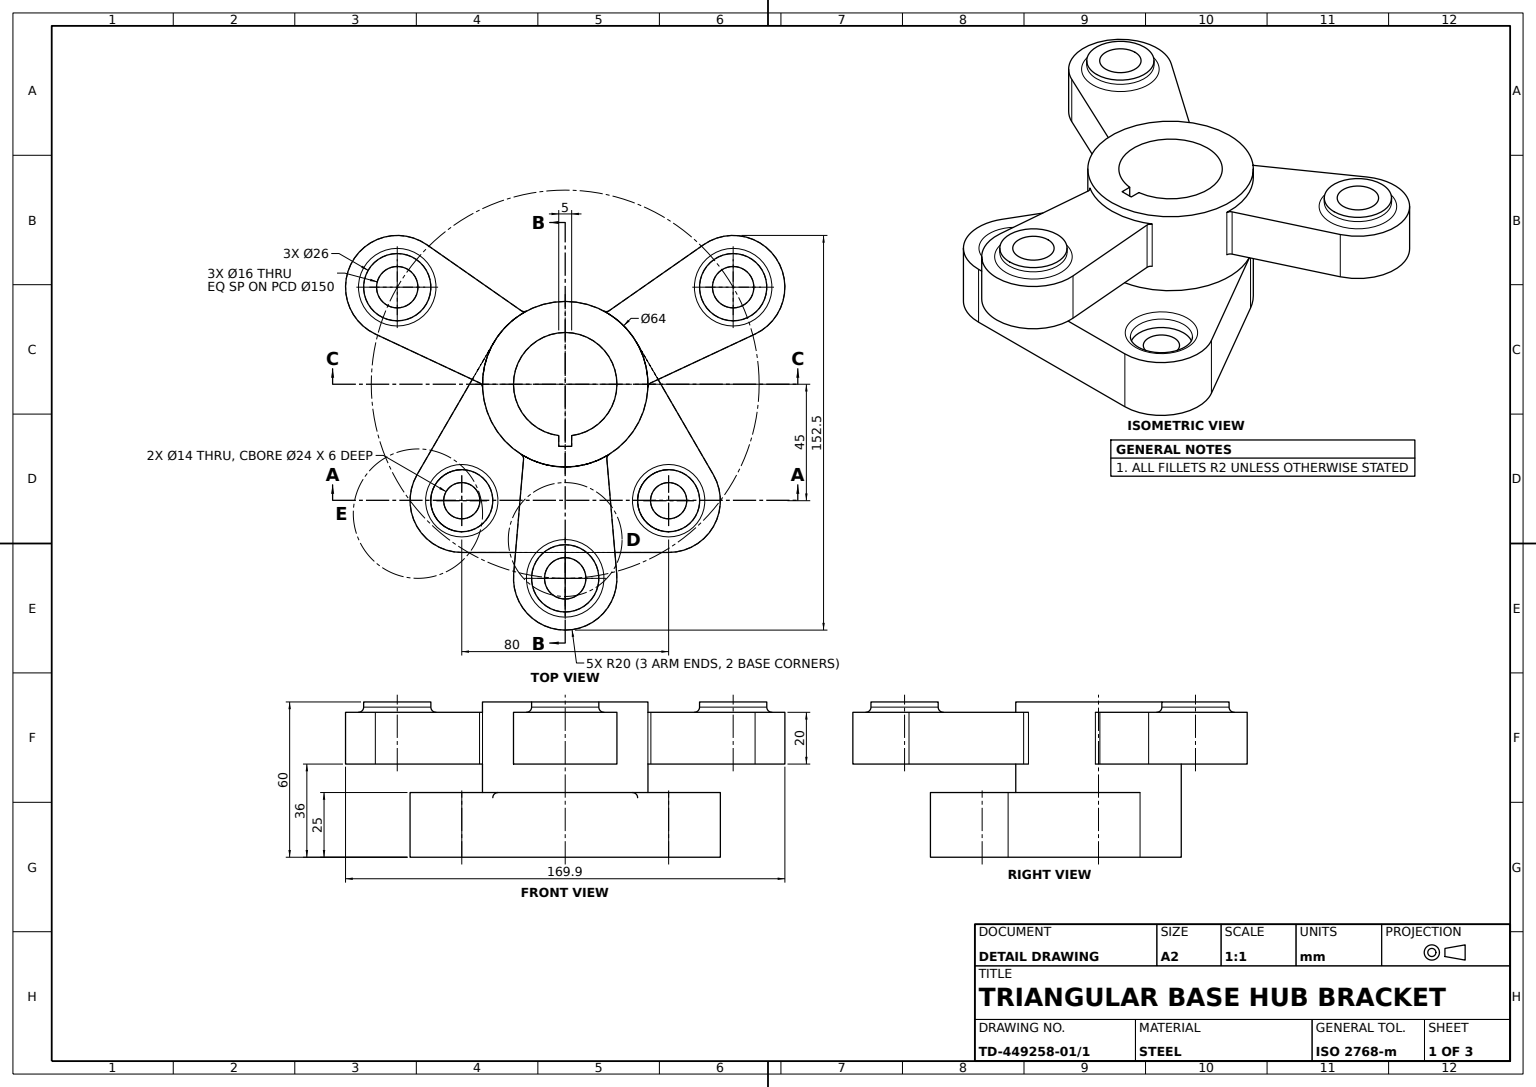
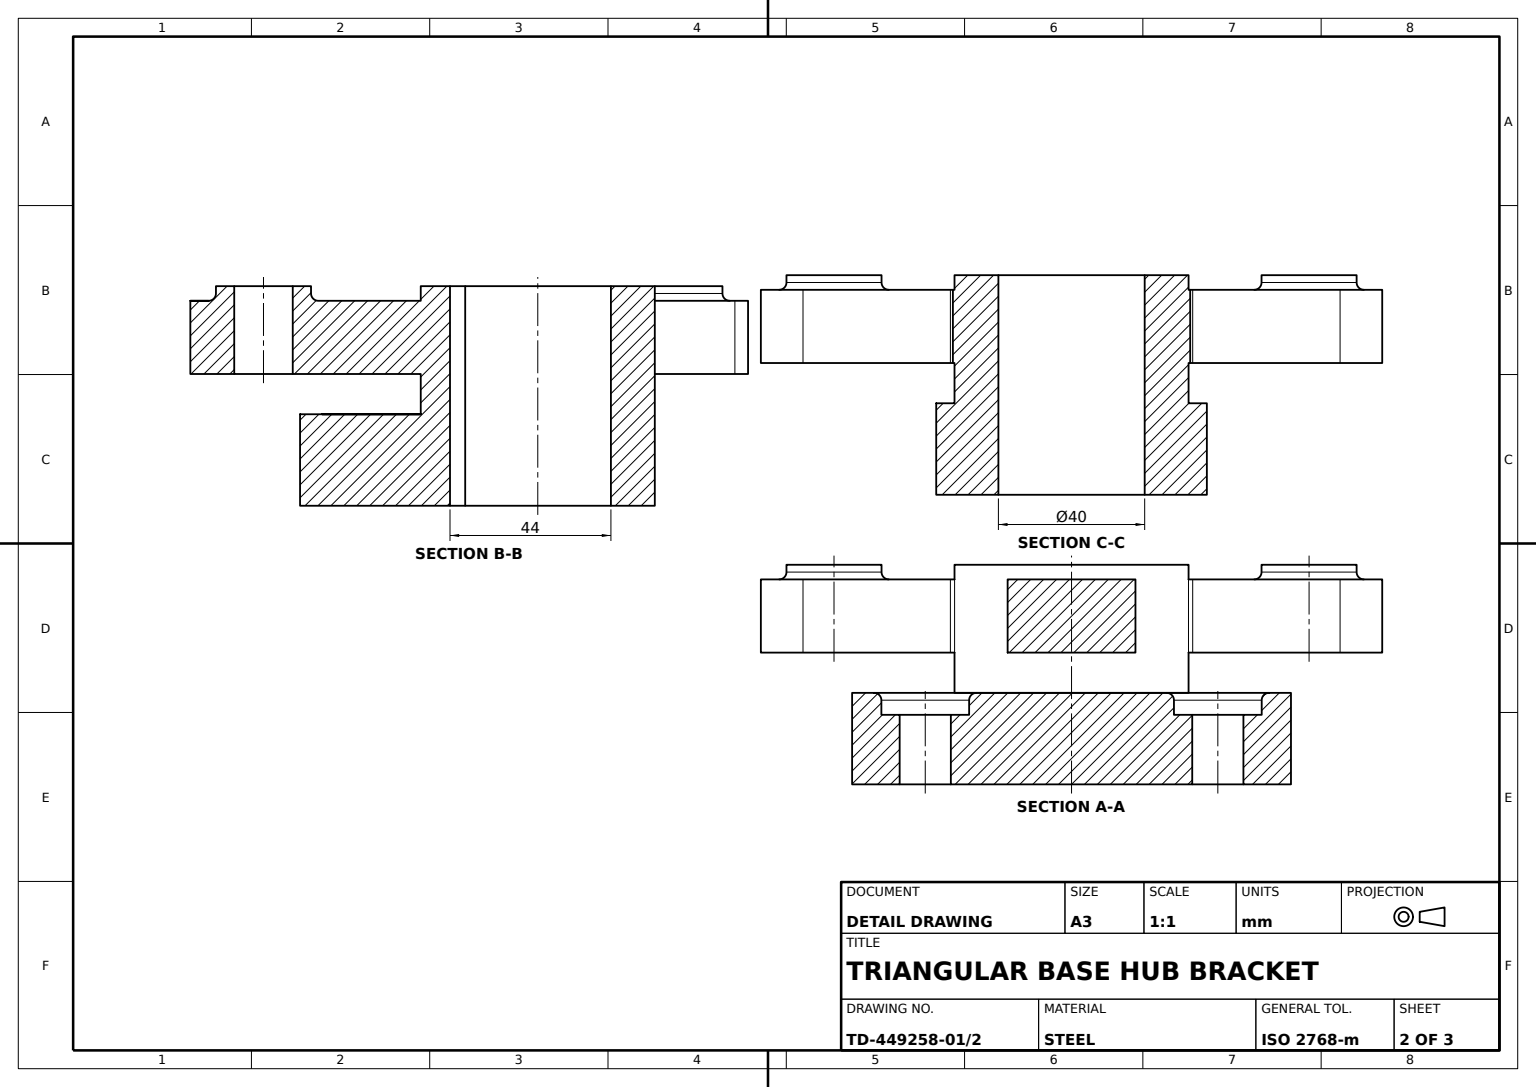
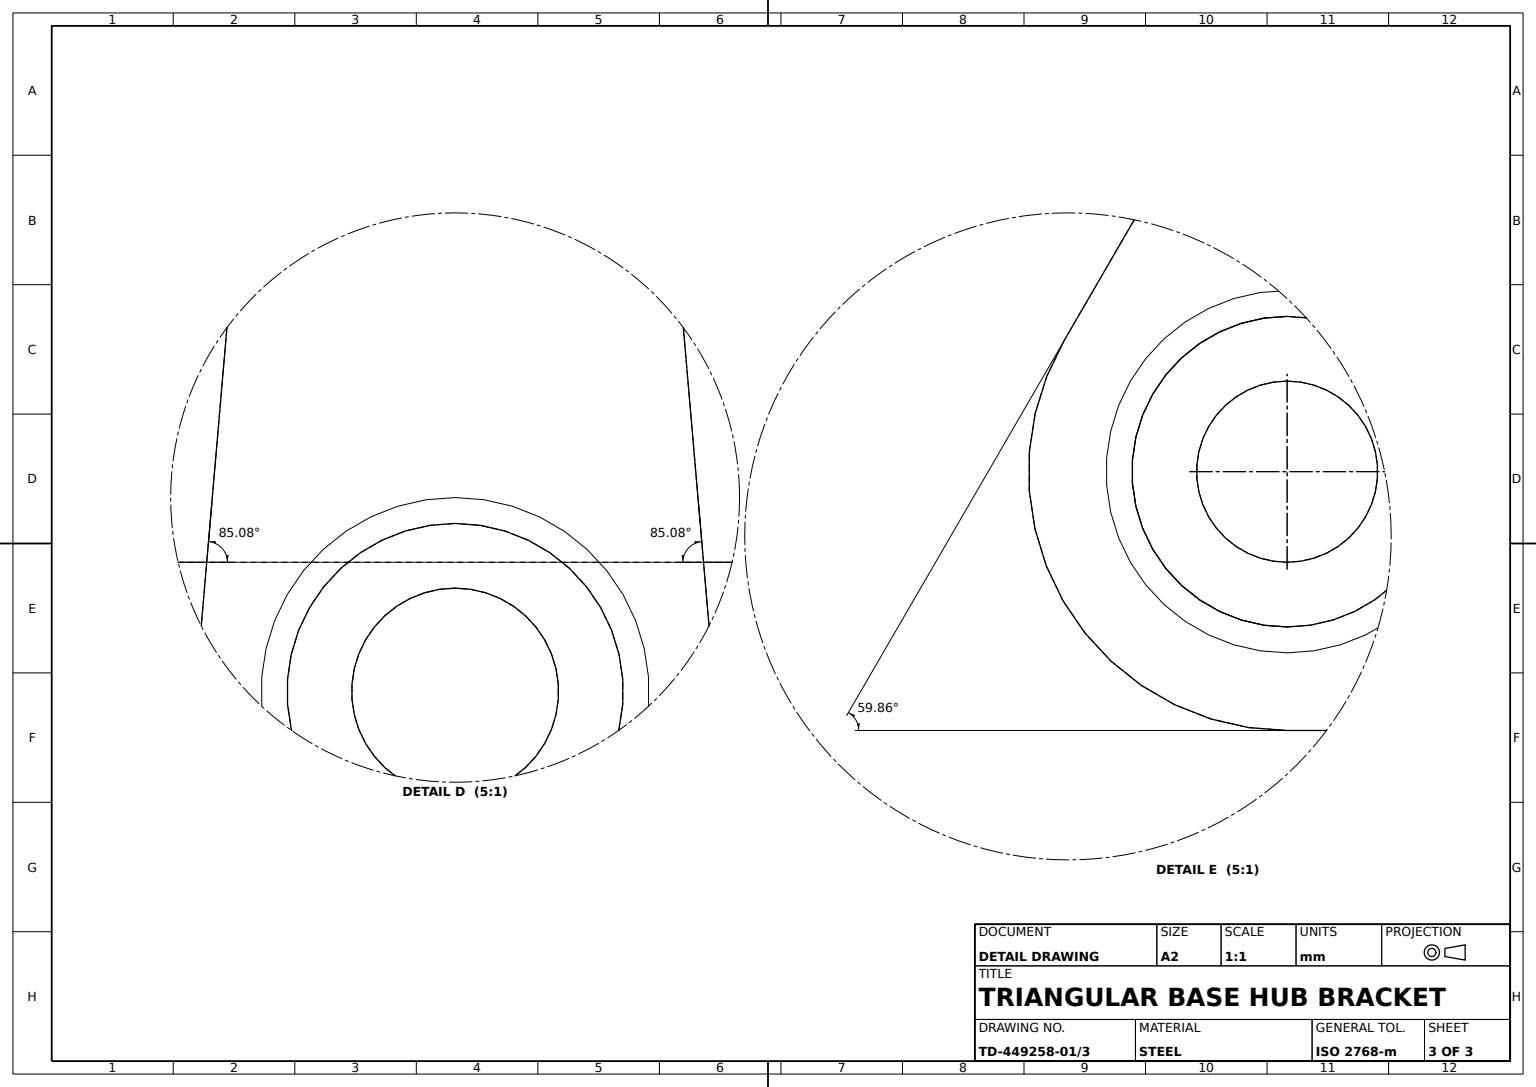
solid
v1 (73.428232,36,-19.385037)
v2 (73.428232,56,-19.385037)
e1 v1 v2 LINE
v3 (33.128128,56,-0.527872)
e2 v3 v2 LINE
v4 (33.128128,36,-0.527872)
e3 v3 v4 LINE
e4 v4 v1 LINE
face PLANE(AX(P(5.747849,36,12.283868),D(0.423816334,0,0.905748152),D(0.905748152,0,-0.423816334))) [e1 -e2 e3 e4]
v5 (-33.128128,36,-0.527872)
v6 (-73.428232,36,-19.385037)
e5 v5 v6 LINE
v7 (-33.128128,56,-0.527872)
e6 v5 v7 LINE
v8 (-73.428232,56,-19.385037)
e7 v7 v8 LINE
e8 v6 v8 LINE
face PLANE(AX(P(-5.747849,36,12.283868),D(0.423816334,0,-0.905748152),D(-0.905748152,0,-0.423816334))) rev [-e5 e6 e7 -e8]
v9 (-2.5,60,24)
v10 (-2.5,0,24)
e9 v9 v10 LINE
v11 (2.5,60,24)
e10 v11 v9 LINE
v12 (2.5,0,24)
e11 v11 v12 LINE
e12 v10 v12 LINE
face PLANE(AX(P(2.5,60,24),D(0,0,1),D(1,0,0))) rev [-e9 -e10 e11 -e12]
v13 (64.951905,58,-50.5)
v14 (64.951905,58,-24.5)
e13 v13 v14 CIRCLE(AX(P(64.951905,58,-37.5),D(0,1,0),D(0,0,1)),13)
v15 (64.951905,56,-52.5)
e14 v13 v15 CIRCLE(AX(P(64.951905,58,-52.5),D(1,0,0),D(0,0,-1)),2)
v16 (64.951905,56,-22.5)
e15 v16 v15 CIRCLE(AX(P(64.951905,56,-37.5),D(0,-1,0),D(0,0,1)),15)
e16 v14 v16 CIRCLE(AX(P(64.951905,58,-22.5),D(-1,0,0),D(0,0,1)),2)
face TORUS(AX(P(64.951905,58,-37.5),D(0,1,0),D(0,0,1)),15,2) rev [-e13 e14 -e15 -e16]
v17 (-64.951905,58,-24.5)
v18 (-64.951905,56,-22.5)
e17 v17 v18 CIRCLE(AX(P(-64.951905,58,-22.5),D(-1,0,0),D(0,0,1)),2)
v19 (-64.951905,58,-50.5)
e18 v19 v17 CIRCLE(AX(P(-64.951905,58,-37.5),D(0,1,0),D(0,0,1)),13)
v20 (-64.951905,56,-52.5)
e19 v19 v20 CIRCLE(AX(P(-64.951905,58,-52.5),D(1,0,0),D(0,0,-1)),2)
e20 v18 v20 CIRCLE(AX(P(-64.951905,56,-37.5),D(0,-1,0),D(0,0,1)),15)
face TORUS(AX(P(-64.951905,58,-37.5),D(0,1,0),D(0,0,1)),15,2) rev [-e17 -e18 e19 -e20]
v21 (0,0,-20)
v22 (-2.5,0,19.843135)
e21 v21 v22 CIRCLE(AX(P(0,0,0),D(0,1,0),D(0,0,1)),20)
v23 (0,60,-20)
e22 v23 v21 LINE
v24 (-2.5,60,19.843135)
e23 v23 v24 CIRCLE(AX(P(0,60,0),D(0,1,0),D(0,0,1)),20)
e24 v24 v22 LINE
face CYL(AX(P(0,60,0),D(0,-1,0),D(0,0,-1)),20) rev [-e21 -e22 e23 e24]
v25 (64.951905,36,-29.5)
v26 (64.951905,36,-45.5)
e25 v25 v26 CIRCLE(AX(P(64.951905,36,-37.5),D(0,1,0),D(0,0,1)),8)
e26 v26 v25 CIRCLE(AX(P(64.951905,36,-37.5),D(0,1,0),D(0,0,1)),8)
v27 (31.977186,36,1.208117)
e27 v4 v27 CIRCLE(AX(P(33.975761,36,1.283624),D(0,1,0),D(0,0,1)),2)
v28 (14.942333,36,-28.297114)
e28 v27 v28 CIRCLE(AX(P(0,36,0),D(0,1,0),D(0,0,1)),32)
v29 (17.021214,36,-28.425864)
e29 v28 v29 CIRCLE(AX(P(15.876229,36,-30.065684),D(0,1,0),D(0,0,1)),2)
v30 (53.50205,36,-53.898196)
e30 v29 v30 LINE
e31 v1 v30 CIRCLE(AX(P(64.951905,36,-37.5),D(0,1,0),D(0,0,1)),20)
face PLANE(AX(P(0,36,0),D(0,1,0),D(0,0,1))) rev [e25 e26] [e27 e28 e29 e30 -e31 -e4]
v31 (64.951905,60,-50.5)
v32 (64.951905,60,-24.5)
e32 v31 v32 CIRCLE(AX(P(64.951905,60,-37.5),D(0,1,0),D(0,0,1)),13)
e33 v32 v31 CIRCLE(AX(P(64.951905,60,-37.5),D(0,1,0),D(0,0,1)),13)
v33 (64.951905,60,-29.5)
v34 (64.951905,60,-45.5)
e34 v33 v34 CIRCLE(AX(P(64.951905,60,-37.5),D(0,1,0),D(0,0,1)),8)
e35 v34 v33 CIRCLE(AX(P(64.951905,60,-37.5),D(0,1,0),D(0,0,1)),8)
face PLANE(AX(P(0,60,0),D(0,1,0),D(0,0,1))) [e32 e33] [-e34 -e35]
v35 (0,36,83)
v36 (0,36,67)
e36 v35 v36 CIRCLE(AX(P(0,36,75),D(0,1,0),D(-0.866025404,0,-0.5)),8)
v37 (0,60,83)
e37 v35 v37 LINE
v38 (0,60,67)
e38 v37 v38 CIRCLE(AX(P(0,60,75),D(0,1,0),D(-0.866025404,0,-0.5)),8)
e39 v36 v38 LINE
face CYL(AX(P(0,36,75),D(0,1,0),D(0,0,1)),8) rev [-e36 e37 e38 -e39]
e40 v14 v32 LINE
e41 v13 v31 LINE
face CYL(AX(P(64.951905,36,-37.5),D(0,1,0),D(0,0,1)),13) [e40 -e32 -e41 e13]
v39 (40,25,65)
v40 (40,0,65)
e42 v39 v40 LINE
v41 (57.296552,0,34.958621)
e43 v40 v41 CIRCLE(AX(P(40,0,45),D(0,1,0),D(0,0,1)),20)
v42 (57.296552,25,34.958621)
e44 v42 v41 LINE
e45 v39 v42 CIRCLE(AX(P(40,25,45),D(0,1,0),D(0,0,1)),20)
face CYL(AX(P(40,25,45),D(0,-1,0),D(0,0,-1)),20) [e42 e43 -e44 -e45]
v43 (19.926182,36,73.283233)
v44 (19.926182,56,73.283233)
e46 v43 v44 LINE
v45 (0,56,95)
e47 v45 v44 CIRCLE(AX(P(0,56,75),D(0,1,0),D(-0.866025404,0,-0.5)),20)
v46 (0,36,95)
e48 v46 v45 LINE
e49 v46 v43 CIRCLE(AX(P(0,36,75),D(0,1,0),D(-0.866025404,0,-0.5)),20)
face CYL(AX(P(0,36,75),D(0,1,0),D(0,0,1)),20) [e46 -e47 -e48 e49]
v47 (-57.296552,0,34.958621)
v48 (-27.674483,0,-16.066207)
e50 v47 v48 LINE
v49 (-57.296552,25,34.958621)
e51 v49 v47 LINE
v50 (-27.674483,25,-16.066207)
e52 v49 v50 LINE
e53 v50 v48 LINE
face PLANE(AX(P(-27.674483,25,-16.066207),D(-0.864827586,0,-0.502068966),D(-0.502068966,0,0.864827586))) [-e50 -e51 e52 e53]
v51 (-64.951905,60,-45.5)
v52 (-64.951905,60,-29.5)
e54 v51 v52 CIRCLE(AX(P(-64.951905,60,-37.5),D(0,1,0),D(0.866025404,0,-0.5)),8)
e55 v52 v51 CIRCLE(AX(P(-64.951905,60,-37.5),D(0,1,0),D(0.866025404,0,-0.5)),8)
v53 (-64.951905,60,-50.5)
v54 (-64.951905,60,-24.5)
e56 v53 v54 CIRCLE(AX(P(-64.951905,60,-37.5),D(0,1,0),D(0.866025404,0,-0.5)),13)
e57 v54 v53 CIRCLE(AX(P(-64.951905,60,-37.5),D(0,1,0),D(0.866025404,0,-0.5)),13)
face PLANE(AX(P(0,60,0),D(0,1,0),D(0.866025404,0,-0.5))) [-e54 -e55] [e56 e57]
v55 (0,60,62)
v56 (0,60,88)
e58 v55 v56 CIRCLE(AX(P(0,60,75),D(0,1,0),D(-0.866025404,0,-0.5)),13)
v57 (0,58,62)
e59 v57 v55 LINE
v58 (0,58,88)
e60 v57 v58 CIRCLE(AX(P(0,58,75),D(0,1,0),D(0,0,1)),13)
e61 v58 v56 LINE
face CYL(AX(P(0,36,75),D(0,1,0),D(0,0,1)),13) [-e58 -e59 e60 e61]
v59 (-40,19,57)
v60 (-40,23,57)
e62 v59 v60 LINE
v61 (-40,23,33)
e63 v60 v61 CIRCLE(AX(P(-40,23,45),D(0,1,0),D(0,0,1)),12)
v62 (-40,19,33)
e64 v62 v61 LINE
e65 v59 v62 CIRCLE(AX(P(-40,19,45),D(0,1,0),D(0,0,1)),12)
face CYL(AX(P(-40,25,45),D(0,1,0),D(0,0,1)),12) rev [e62 e63 -e64 -e65]
v63 (40,19,33)
v64 (40,23,33)
e66 v63 v64 LINE
v65 (40,23,57)
e67 v64 v65 CIRCLE(AX(P(40,23,45),D(0,1,0),D(0,0,1)),12)
v66 (40,19,57)
e68 v66 v65 LINE
e69 v63 v66 CIRCLE(AX(P(40,19,45),D(0,1,0),D(0,0,1)),12)
face CYL(AX(P(40,25,45),D(0,1,0),D(0,0,1)),12) rev [e66 e67 -e68 -e69]
v67 (-17.021214,56,-28.425864)
v68 (-53.50205,56,-53.898196)
e70 v67 v68 LINE
v69 (-17.021214,36,-28.425864)
e71 v67 v69 LINE
v70 (-53.50205,36,-53.898196)
e72 v69 v70 LINE
e73 v70 v68 LINE
face PLANE(AX(P(7.764217,36,-11.119717),D(0.572492742,0,-0.819909788),D(-0.819909788,0,-0.572492742))) [-e70 e71 e72 e73]
v71 (16.106913,56,28.953736)
v72 (17.034853,56,27.088997)
e74 v71 v72 CIRCLE(AX(P(18.099532,56,28.78206),D(0,-1,0),D(0,0,1)),2)
v73 (16.106913,36,28.953736)
e75 v73 v71 LINE
v74 (17.034853,36,27.088997)
e76 v74 v73 CIRCLE(AX(P(18.099532,36,28.78206),D(0,1,0),D(0,0,1)),2)
e77 v72 v74 LINE
face CYL(AX(P(18.099532,25,28.78206),D(0,-1,0),D(0,0,-1)),2) rev [-e74 -e75 -e76 -e77]
e78 v38 v37 CIRCLE(AX(P(0,60,75),D(0,1,0),D(-0.866025404,0,-0.5)),8)
e79 v36 v35 CIRCLE(AX(P(0,36,75),D(0,1,0),D(-0.866025404,0,-0.5)),8)
face CYL(AX(P(0,36,75),D(0,1,0),D(0,0,1)),8) rev [e39 e78 -e37 -e79]
e80 v58 v57 CIRCLE(AX(P(0,58,75),D(0,1,0),D(0,0,1)),13)
v75 (0,56,90)
e81 v58 v75 CIRCLE(AX(P(0,58,90),D(-1,0,0),D(0,0,1)),2)
v76 (0,56,60)
e82 v76 v75 CIRCLE(AX(P(0,56,75),D(0,-1,0),D(0,0,1)),15)
e83 v57 v76 CIRCLE(AX(P(0,58,60),D(1,0,0),D(0,0,-1)),2)
face TORUS(AX(P(0,58,75),D(0,1,0),D(0,0,1)),15,2) rev [-e80 e81 -e82 -e83]
v77 (53.50205,56,-53.898196)
e84 v2 v77 CIRCLE(AX(P(64.951905,56,-37.5),D(0,1,0),D(0,0,1)),20)
e85 v30 v77 LINE
face CYL(AX(P(64.951905,36,-37.5),D(0,1,0),D(0,0,1)),20) [-e84 -e1 e31 e85]
v78 (-40,0,65)
e86 v78 v47 CIRCLE(AX(P(-40,0,45),D(0,-1,0),D(0,0,1)),20)
v79 (-40,25,65)
e87 v79 v78 LINE
e88 v79 v49 CIRCLE(AX(P(-40,25,45),D(0,-1,0),D(0,0,1)),20)
face CYL(AX(P(-40,25,45),D(0,-1,0),D(0,0,-1)),20) [e51 -e86 -e87 e88]
e89 v19 v53 LINE
e90 v17 v54 LINE
face CYL(AX(P(-64.951905,36,-37.5),D(0,1,0),D(0,0,1)),13) [-e56 -e89 e18 e90]
v80 (-31.977186,36,1.208117)
e91 v80 v5 CIRCLE(AX(P(-33.975761,36,1.283624),D(0,1,0),D(0,0,1)),2)
v81 (-31.977186,56,1.208117)
e92 v81 v80 LINE
e93 v7 v81 CIRCLE(AX(P(-33.975761,56,1.283624),D(0,-1,0),D(0,0,1)),2)
face CYL(AX(P(-33.975761,25,1.283624),D(0,-1,0),D(0,0,-1)),2) rev [-e91 -e92 -e93 -e6]
v82 (-14.942333,56,-28.297114)
e94 v82 v81 CIRCLE(AX(P(0,56,0),D(0,1,0),D(0.866025404,0,-0.5)),32)
v83 (-14.942333,36,-28.297114)
e95 v83 v80 CIRCLE(AX(P(0,36,0),D(0,1,0),D(0.866025404,0,-0.5)),32)
e96 v83 v82 LINE
v84 (0,25,32)
e97 v84 v50 CIRCLE(AX(P(0,25,0),D(0,-1,0),D(0,0,1)),32)
v85 (0,36,32)
e98 v85 v84 LINE
v86 (-17.034853,36,27.088997)
e99 v86 v85 CIRCLE(AX(P(0,36,0),D(0,1,0),D(-0.866025404,0,-0.5)),32)
v87 (-17.034853,56,27.088997)
e100 v86 v87 LINE
v88 (0,56,32)
e101 v87 v88 CIRCLE(AX(P(0,56,0),D(0,1,0),D(-0.866025404,0,-0.5)),32)
v89 (0,60,32)
e102 v89 v88 LINE
v90 (0,60,-32)
e103 v90 v89 CIRCLE(AX(P(0,60,0),D(0,1,0),D(0,0,1)),32)
v91 (0,0,-32)
e104 v90 v91 LINE
e105 v91 v48 CIRCLE(AX(P(0,0,0),D(0,1,0),D(0,0,1)),32)
face CYL(AX(P(0,25,0),D(0,-1,0),D(0,0,-1)),32) [e94 e92 -e95 e96] [-e97 -e98 -e99 e100 e101 -e102 -e103 e104 e105 -e53]
v92 (40,25,59)
v93 (40,25,31)
e106 v92 v93 CIRCLE(AX(P(40,25,45),D(0,-1,0),D(0,0,1)),14)
e107 v93 v92 CIRCLE(AX(P(40,25,45),D(0,-1,0),D(0,0,1)),14)
v94 (-40,25,31)
v95 (-40,25,59)
e108 v94 v95 CIRCLE(AX(P(-40,25,45),D(0,-1,0),D(0,0,1)),14)
e109 v95 v94 CIRCLE(AX(P(-40,25,45),D(0,-1,0),D(0,0,1)),14)
v96 (27.674483,25,-16.066207)
e110 v96 v84 CIRCLE(AX(P(0,25,0),D(0,-1,0),D(0,0,1)),32)
e111 v39 v79 LINE
e112 v42 v96 LINE
face PLANE(AX(P(0,25,0),D(0,1,0),D(0,0,1))) [e106 e107] [e108 e109] [e110 e97 -e52 -e88 -e111 e45 e112]
e113 v89 v90 CIRCLE(AX(P(0,60,0),D(0,1,0),D(0,0,1)),32)
v97 (2.5,60,19.843135)
e114 v97 v23 CIRCLE(AX(P(0,60,0),D(0,1,0),D(0,0,1)),20)
e115 v97 v11 LINE
e116 v24 v9 LINE
face PLANE(AX(P(0,60,0),D(0,1,0),D(0,0,1))) [e103 e113] [-e23 -e114 e115 e10 -e116]
e117 v14 v13 CIRCLE(AX(P(64.951905,58,-37.5),D(0,1,0),D(0,0,1)),13)
face CYL(AX(P(64.951905,36,-37.5),D(0,1,0),D(0,0,1)),13) [-e33 -e40 e117 e41]
v98 (-19.926182,56,73.283233)
e118 v98 v45 CIRCLE(AX(P(0,56,75),D(0,1,0),D(-0.866025404,0,-0.5)),20)
v99 (-19.926182,36,73.283233)
e119 v99 v98 LINE
e120 v99 v46 CIRCLE(AX(P(0,36,75),D(0,1,0),D(-0.866025404,0,-0.5)),20)
face CYL(AX(P(0,36,75),D(0,1,0),D(0,0,1)),20) [-e118 -e119 e120 e48]
e121 v40 v78 LINE
face PLANE(AX(P(0,25,65),D(0,0,1),D(1,0,0))) [e111 e87 -e121 -e42]
v100 (-40,0,38)
v101 (-40,0,52)
e122 v100 v101 CIRCLE(AX(P(-40,0,45),D(0,1,0),D(0,0,1)),7)
v102 (-40,19,38)
e123 v100 v102 LINE
v103 (-40,19,52)
e124 v102 v103 CIRCLE(AX(P(-40,19,45),D(0,1,0),D(0,0,1)),7)
e125 v101 v103 LINE
face CYL(AX(P(-40,25,45),D(0,1,0),D(0,0,1)),7) rev [-e122 e123 e124 -e125]
e126 v17 v19 CIRCLE(AX(P(-64.951905,58,-37.5),D(0,1,0),D(0,0,1)),13)
face CYL(AX(P(-64.951905,36,-37.5),D(0,1,0),D(0,0,1)),13) [-e90 e126 e89 -e57]
v104 (31.977186,56,1.208117)
e127 v104 v3 CIRCLE(AX(P(33.975761,56,1.283624),D(0,-1,0),D(0,0,1)),2)
e128 v27 v104 LINE
face CYL(AX(P(33.975761,25,1.283624),D(0,-1,0),D(0,0,-1)),2) rev [-e27 -e3 -e127 -e128]
e129 v101 v100 CIRCLE(AX(P(-40,0,45),D(0,1,0),D(0,0,1)),7)
v105 (40,0,38)
v106 (40,0,52)
e130 v105 v106 CIRCLE(AX(P(40,0,45),D(0,1,0),D(0,0,1)),7)
e131 v106 v105 CIRCLE(AX(P(40,0,45),D(0,1,0),D(0,0,1)),7)
v107 (27.674483,0,-16.066207)
e132 v107 v91 CIRCLE(AX(P(0,0,0),D(0,1,0),D(0,0,1)),32)
e133 v41 v107 LINE
e134 v22 v10 LINE
v108 (2.5,0,19.843135)
e135 v12 v108 LINE
e136 v108 v21 CIRCLE(AX(P(0,0,0),D(0,1,0),D(0,0,1)),20)
face PLANE(AX(P(0,0,0),D(0,1,0),D(0,0,1))) rev [e122 e129] [e130 e131] [-e132 -e133 -e43 e121 e86 e50 -e105] [e134 e12 e135 e136 e21]
e137 v70 v6 CIRCLE(AX(P(-64.951905,36,-37.5),D(0,1,0),D(0.866025404,0,-0.5)),20)
e138 v69 v83 CIRCLE(AX(P(-15.876229,36,-30.065684),D(0,1,0),D(0,0,1)),2)
v109 (-64.951905,36,-45.5)
v110 (-64.951905,36,-29.5)
e139 v109 v110 CIRCLE(AX(P(-64.951905,36,-37.5),D(0,1,0),D(0.866025404,0,-0.5)),8)
e140 v110 v109 CIRCLE(AX(P(-64.951905,36,-37.5),D(0,1,0),D(0.866025404,0,-0.5)),8)
face PLANE(AX(P(0,36,0),D(0,1,0),D(0.866025404,0,-0.5))) rev [e5 -e137 -e72 e138 e95 e91] [e139 e140]
face PLANE(AX(P(-2.5,60,19.843135),D(1,0,0),D(0,0,-1))) [-e24 e116 e9 -e134]
e141 v75 v76 CIRCLE(AX(P(0,56,75),D(0,-1,0),D(0,0,1)),15)
face TORUS(AX(P(0,58,75),D(0,1,0),D(0,0,1)),15,2) rev [-e60 e83 -e141 -e81]
e142 v103 v102 CIRCLE(AX(P(-40,19,45),D(0,1,0),D(0,0,1)),7)
face CYL(AX(P(-40,25,45),D(0,1,0),D(0,0,1)),7) rev [e142 -e123 -e129 e125]
e143 v92 v65 CIRCLE(AX(P(40,23,59),D(-1,0,0),D(0,0,1)),2)
e144 v93 v64 CIRCLE(AX(P(40,23,31),D(1,0,0),D(0,0,-1)),2)
face TORUS(AX(P(40,23,45),D(0,1,0),D(0,0,1)),14,2) [e143 -e67 -e144 -e106]
e145 v95 v60 CIRCLE(AX(P(-40,23,59),D(-1,0,0),D(0,0,1)),2)
e146 v61 v60 CIRCLE(AX(P(-40,23,45),D(0,1,0),D(0,0,1)),12)
e147 v94 v61 CIRCLE(AX(P(-40,23,31),D(1,0,0),D(0,0,-1)),2)
face TORUS(AX(P(-40,23,45),D(0,1,0),D(0,0,1)),14,2) [e145 -e146 -e147 -e109]
v111 (14.942333,56,-28.297114)
e148 v111 v28 LINE
v112 (17.021214,56,-28.425864)
e149 v112 v111 CIRCLE(AX(P(15.876229,56,-30.065684),D(0,-1,0),D(0,0,1)),2)
e150 v29 v112 LINE
face CYL(AX(P(15.876229,25,-30.065684),D(0,-1,0),D(0,0,-1)),2) rev [-e148 -e149 -e150 -e29]
e151 v97 v108 LINE
face CYL(AX(P(0,60,0),D(0,-1,0),D(0,0,-1)),20) rev [e22 -e136 -e151 e114]
e152 v82 v67 CIRCLE(AX(P(-15.876229,56,-30.065684),D(0,-1,0),D(0,0,1)),2)
face CYL(AX(P(-15.876229,25,-30.065684),D(0,-1,0),D(0,0,-1)),2) rev [-e138 -e71 -e152 -e96]
e153 v15 v16 CIRCLE(AX(P(64.951905,56,-37.5),D(0,-1,0),D(0,0,1)),15)
face TORUS(AX(P(64.951905,58,-37.5),D(0,1,0),D(0,0,1)),15,2) rev [-e117 e16 -e153 -e14]
e154 v62 v59 CIRCLE(AX(P(-40,19,45),D(0,1,0),D(0,0,1)),12)
face CYL(AX(P(-40,25,45),D(0,1,0),D(0,0,1)),12) rev [e146 -e62 -e154 e64]
e155 v96 v107 LINE
face PLANE(AX(P(27.674483,25,-16.066207),D(-0.864827586,0,0.502068966),D(0.502068966,0,0.864827586))) rev [e133 -e155 -e112 e44]
v113 (-16.106913,36,28.953736)
e156 v113 v99 LINE
v114 (-16.106913,56,28.953736)
e157 v114 v98 LINE
e158 v114 v113 LINE
face PLANE(AX(P(-13.512066,36,-1.16415),D(-0.996309076,0,-0.085838364),D(-0.085838364,0,0.996309076))) [e156 e119 -e157 e158]
v115 (40,19,38)
e159 v105 v115 LINE
v116 (40,19,52)
e160 v115 v116 CIRCLE(AX(P(40,19,45),D(0,1,0),D(0,0,1)),7)
e161 v106 v116 LINE
face CYL(AX(P(40,25,45),D(0,1,0),D(0,0,1)),7) rev [-e130 e159 e160 -e161]
e162 v112 v77 LINE
face PLANE(AX(P(-7.764217,36,-11.119717),D(0.572492742,0,0.819909788),D(0.819909788,0,-0.572492742))) rev [-e30 e150 e162 -e85]
e163 v109 v51 LINE
e164 v110 v52 LINE
face CYL(AX(P(-64.951905,36,-37.5),D(0,1,0),D(0,0,1)),8) rev [e163 e54 -e164 -e139]
e165 v20 v18 CIRCLE(AX(P(-64.951905,56,-37.5),D(0,-1,0),D(0,0,1)),15)
face TORUS(AX(P(-64.951905,58,-37.5),D(0,1,0),D(0,0,1)),15,2) rev [-e19 -e126 e17 -e165]
e166 v26 v34 LINE
e167 v25 v33 LINE
face CYL(AX(P(64.951905,36,-37.5),D(0,1,0),D(0,0,1)),8) rev [-e166 -e25 e167 e34]
face TORUS(AX(P(-40,23,45),D(0,1,0),D(0,0,1)),14,2) [-e145 -e108 e147 -e63]
e168 v116 v115 CIRCLE(AX(P(40,19,45),D(0,1,0),D(0,0,1)),7)
face CYL(AX(P(40,25,45),D(0,1,0),D(0,0,1)),7) rev [-e159 -e131 e161 e168]
e169 v68 v8 CIRCLE(AX(P(-64.951905,56,-37.5),D(0,1,0),D(0.866025404,0,-0.5)),20)
face CYL(AX(P(-64.951905,36,-37.5),D(0,1,0),D(0,0,1)),20) [-e169 -e73 e137 e8]
e170 v71 v44 LINE
e171 v88 v72 CIRCLE(AX(P(0,56,0),D(0,1,0),D(-0.866025404,0,-0.5)),32)
e172 v87 v114 CIRCLE(AX(P(-18.099532,56,28.78206),D(0,-1,0),D(0,0,1)),2)
face PLANE(AX(P(0,56,0),D(0,1,0),D(-0.866025404,0,-0.5))) [e82 e141] [e157 e118 e47 -e170 e74 -e171 -e101 e172]
e173 v56 v55 CIRCLE(AX(P(0,60,75),D(0,1,0),D(-0.866025404,0,-0.5)),13)
face PLANE(AX(P(0,60,0),D(0,1,0),D(-0.866025404,0,-0.5))) [e173 e58] [-e38 -e78]
face CYL(AX(P(0,36,75),D(0,1,0),D(0,0,1)),13) [-e61 e80 e59 -e173]
e174 v104 v111 CIRCLE(AX(P(0,56,0),D(0,1,0),D(0,0,1)),32)
face PLANE(AX(P(0,56,0),D(0,1,0),D(0,0,1))) [e153 e15] [e127 e2 e84 -e162 e149 -e174]
e175 v65 v64 CIRCLE(AX(P(40,23,45),D(0,1,0),D(0,0,1)),12)
e176 v66 v63 CIRCLE(AX(P(40,19,45),D(0,1,0),D(0,0,1)),12)
face CYL(AX(P(40,25,45),D(0,1,0),D(0,0,1)),12) rev [e175 -e66 -e176 e68]
face PLANE(AX(P(47,19,45),D(0,-1,0),D(0,0,-1))) rev [e176 e69] [-e160 -e168]
e177 v113 v86 CIRCLE(AX(P(-18.099532,36,28.78206),D(0,1,0),D(0,0,1)),2)
face CYL(AX(P(-18.099532,25,28.78206),D(0,-1,0),D(0,0,-1)),2) rev [-e177 -e158 -e172 -e100]
e178 v73 v43 LINE
face PLANE(AX(P(13.512066,36,-1.16415),D(-0.996309076,0,0.085838364),D(0.085838364,0,0.996309076))) rev [-e46 -e178 e75 e170]
face PLANE(AX(P(-33,19,45),D(0,-1,0),D(0,0,-1))) rev [e154 e65] [-e142 -e124]
face PLANE(AX(P(2.5,60,19.843135),D(1,0,0),D(0,0,-1))) rev [e151 -e135 -e11 -e115]
e179 v85 v74 CIRCLE(AX(P(0,36,0),D(0,1,0),D(-0.866025404,0,-0.5)),32)
face PLANE(AX(P(0,36,0),D(0,1,0),D(-0.866025404,0,-0.5))) rev [-e120 -e156 e177 e99 e179 e76 e178 -e49] [e36 e79]
face TORUS(AX(P(40,23,45),D(0,1,0),D(0,0,1)),14,2) [-e143 -e107 e144 -e175]
face CYL(AX(P(-64.951905,36,-37.5),D(0,1,0),D(0,0,1)),8) rev [e164 e55 -e163 -e140]
face CYL(AX(P(64.951905,36,-37.5),D(0,1,0),D(0,0,1)),8) rev [-e26 e166 e35 -e167]
face PLANE(AX(P(0,56,0),D(0,1,0),D(0.866025404,0,-0.5))) [e70 e169 -e7 e93 -e94 e152] [e165 e20]
face CYL(AX(P(0,25,0),D(0,-1,0),D(0,0,-1)),32) [e128 e174 e148 -e28] [e132 -e104 -e113 e102 e171 e77 -e179 e98 -e110 e155]
